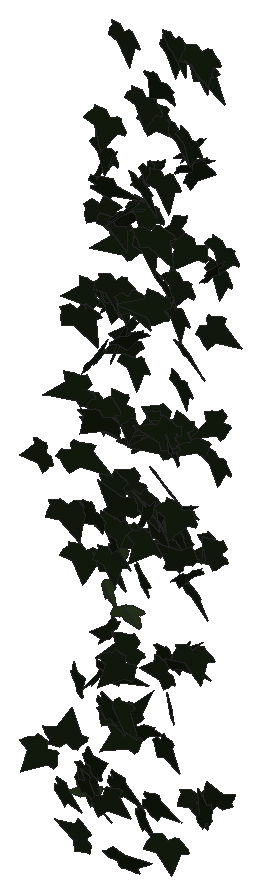
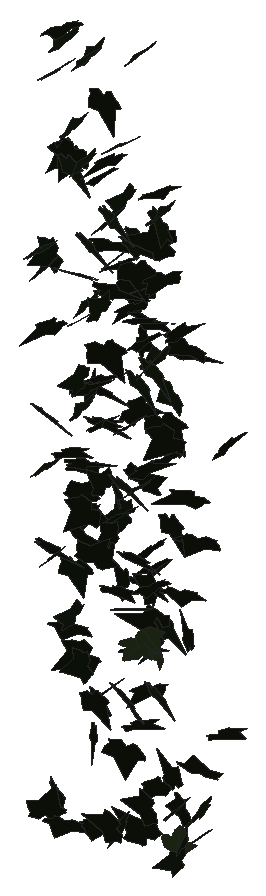
# SketchUp Ruby script. Lengths in inches.
U = 1.inch
M = Sketchup.active_model
def pt(a) = Geom::Point3d.new(a.map { |v| v * U })
def face(e, loops, mat)
  f = e.add_face(loops[0].map { |a| pt(a) })
  loops[1..].each { |l| e.add_face(l.map { |a| pt(a) }).erase! }
  f.material = f.back_material = mat if mat
  f
end
# faces: each face lists its corners as indices into pts; further lists are holes
def faces(e, pts, list, mat = nil) = list.each { |f| face(e, (f[0].is_a?(Array) ? f : [f]).map { |l| l.map { |i| pts[i] } }, mat) }
# xy, xz, yz: faces in a plane at the given z, y or x. An outline is a flat list of corners, or four numbers for a rectangle; further outlines are holes
def ring(l) = l.size == 4 ? [[l[0], l[1]], [l[2], l[1]], [l[2], l[3]], [l[0], l[3]]] : l.each_slice(2).to_a
def flat(e, list, mat, &to3) = list.each { |f| face(e, (f[0].is_a?(Array) ? f : [f]).map { |l| ring(l).map { |u, v| to3.(u, v) } }, mat) }
def xy(e, z, list, mat = nil) = flat(e, list, mat) { |x, y| [x, y, z] }
def xz(e, y, list, mat = nil) = flat(e, list, mat) { |x, z| [x, y, z] }
def yz(e, x, list, mat = nil) = flat(e, list, mat) { |y, z| [x, y, z] }
def lines(e, pts, list) = list.each { |a, b| e.add_line(pt(pts[a]), pt(pts[b])) }
# prism: a flat outline (further loops are holes) pulled along v
def prism(e, loops, v, mat = nil)
  f = face(e, loops, mat); d = Geom::Vector3d.new(v.map { |x| x * U })
  f.pushpull(f.normal.samedirection?(d) ? d.length : -d.length)
end
def box(e, o, s, mat = nil) = prism(e, [[o, [o[0] + s[0], o[1], o[2]], [o[0] + s[0], o[1] + s[1], o[2]], [o[0], o[1] + s[1], o[2]]]], [0, 0, s[2]], mat)
def at(x, y, z, deg = 0) = Geom::Transformation.translation(pt([x, y, z])) * Geom::Transformation.rotation(ORIGIN, Z_AXIS, deg.degrees)
def axes(o, x, y, z) = Geom::Transformation.new([*x, 0, *y, 0, *z, 0, *pt(o).to_a, 1])
def part(name) = M.definitions.add(name)
# library, detail: a bought-in or finely detailed component or shape, given as its bounding box
def library(name, o, s) = part(name).tap { |d| box(d.entities, o, s) }
def detail(e, o, s) = box(e.add_group.entities, o, s)
def put(e, d, t, mat = nil) = e.add_instance(d, t).tap { |i| i.material = mat if mat }
def group(e, t, mat = nil) = e.add_group.tap { |g| g.transformation = t; g.material = mat if mat }.entities
root = M.entities
M.materials.add("1026 AP 7946 SUNNY SIDE UP").color = [254, 231, 186]
M.materials.add("efeu1").color = [18, 25, 13]
M.materials.add("efeu2").color = [43, 57, 29]
c1 = part("ivyleaf_9")
p = [[1.54,2.16,1.25],[1.36,2.04,1.19],[-0.21,0.99,0.68],[-0.71,1.11,0.82],[-0.85,0.86,0.67],[-0.8,0.17,0.21],
  [-0.9,-0.01,0.1],[-0.67,-0.16,-0.02],[-0.08,-0.08,-0.05],[-0.03,-0.6,-0.4],[0.65,-0.88,-0.66],[0.83,-0.6,-0.49],
  [1.29,-0.42,-0.43],[1.8125,-0.07,-0.26],[1.21,0.44,0.15]]
faces(c1.entities,p,[[0,1,2,3,4,5,6,7,8,9,10,11,12,13,14]],"efeu1")
c2 = part("ivyleaf_10")
p = [[0,0.5,-0.03],[-0.0625,2.02,-0.43],[-0.19,2.01,-0.46],[-0.54,1.05,-0.29],[-0.52,0.625,-0.18],[-0.83,0.76,-0.28],
  [-1.16,0.64,-0.33],[-1.15,0.33,-0.24],[-0.77,-0.39,0.02],[-0.3,-0.51,0.16],[0.04,-0.48,0.23],[-0.02,2.01,-0.4375],
  [-0.06,2.01,-0.43],[0.04,-0.49,0.23],[0.67,-0.49,0.14],[1.38,0.36,-0.2],[1.375,0.51,-0.24],[0.81,0.65,-0.19],
  [0.62,0.59,-0.15],[0.6,1.09,-0.28],[0.5,1.23,-0.31]]
faces(c2.entities,p,[[0,1,2,3,4,5,6,7,8,9,10],[11,12,0,13,14,15,16,17,18,19,20]],"efeu2")
put(root,c1,axes([163.08,208.98,294.97],[-0.63448,0.06038,0.18044],[0.28089,0.01865,0.41828],[0.07528,0.43936,-0.03993]),"1026 AP 7946 SUNNY SIDE UP")
put(root,c1,axes([163.05,207.6,308.75],[0.10411,-0.32993,-0.29314],[0.18645,-0.26136,0.34135],[-0.65722,-0.12641,0.0504]),"1026 AP 7946 SUNNY SIDE UP")
put(root,c1,axes([162.83,211.46,318.29],[0.01182,-0.3708,-0.31812],[-0.03173,0.30622,-0.38012],[0.75597,0.01865,-0.01098]),"1026 AP 7946 SUNNY SIDE UP")
put(root,c1,axes([163.41,211.59,314.12],[-0.30515,0.40603,0.05346],[-0.04881,0.04011,-0.46325],[-0.64133,-0.19624,0.00982]),"1026 AP 7946 SUNNY SIDE UP")
put(root,c1,axes([162.99,211.79,322.14],[-0.27864,-0.43252,0.07285],[-0.00325,-0.07809,-0.48116],[0.68975,-0.17509,0.02716]),"1026 AP 7946 SUNNY SIDE UP")
put(root,c2,axes([163.2,210.21,292.14],[-0.48083,-0.24254,-0.10357],[-0.14812,-0.04045,0.40096],[-0.38447,0.31891,-0.02494]),"1026 AP 7946 SUNNY SIDE UP")
put(root,c2,axes([163.27,212.04,302.38],[-0.29776,-0.29187,0.20443],[-0.10278,-0.19419,-0.35667],[0.54686,-0.19542,0.04428]),"1026 AP 7946 SUNNY SIDE UP")
put(root,c1,axes([163.35,210.97,320.28],[0.00242,0.34278,0.33575],[-0.00805,0.32396,-0.3512],[-0.74157,-0.00239,0.00491]),"1026 AP 7946 SUNNY SIDE UP")
put(root,c1,axes([162.9375,209.25,305.52],[-0.29022,-0.31053,-0.2798],[0.24286,0.22181,-0.37051],[0.59955,-0.24016,0.01464]),"1026 AP 7946 SUNNY SIDE UP")
put(root,c1,axes([163.37,210.26,314.9],[-0.23905,-0.11298,0.40638],[-0.41094,-0.29853,-0.19328],[0.49866,-0.30017,0.03553]),"1026 AP 7946 SUNNY SIDE UP")
put(root,c1,axes([162.76,210.6,291.82],[0.50726,-0.26293,0.05987],[0.04536,-0.05876,-0.42818],[0.4215,0.32276,-0.02598]),"1026 AP 7946 SUNNY SIDE UP")
put(root,c1,axes([162.76,209.8125,307.75],[0.17736,-0.21342,-0.40951],[0.28851,0.39487,-0.16296],[0.64629,-0.1177,0.18513]),"1026 AP 7946 SUNNY SIDE UP")
put(root,c1,axes([162.98,210.26,292.22],[0.08539,-0.23069,0.33356],[0.07354,-0.32214,-0.24543],[0.62247,0.0697,-0.01676]),"1026 AP 7946 SUNNY SIDE UP")
put(root,c1,axes([163.07,211.49,314.72],[0.35675,-0.26779,-0.29291],[-0.23182,0.24388,-0.35833],[0.56683,0.26828,0.0378]),"1026 AP 7946 SUNNY SIDE UP")
put(root,c1,axes([163.04,211.53,320.92],[-0.05014,-0.38539,0.28073],[0.01768,-0.27585,-0.39897],[0.74395,-0.01941,0.0284]),"1026 AP 7946 SUNNY SIDE UP")
put(root,c1,axes([163.64,212.34,316.41],[-0.57045,-0.06544,0.26432],[-0.3141,-0.21888,-0.34928],[0.27415,-0.38695,0.14981]),"1026 AP 7946 SUNNY SIDE UP")
put(root,c1,axes([163.68,211.02,299.28],[-0.30723,0.33384,0.12004],[-0.11068,0.09153,-0.3977],[-0.54386,-0.20722,0.01313]),"1026 AP 7946 SUNNY SIDE UP")
put(root,c1,axes([163.15,208.4375,293.17],[0.44463,-0.23051,-0.25194],[-0.24259,0.19299,-0.37205],[0.46778,0.31919,0.04653]),"1026 AP 7946 SUNNY SIDE UP")
put(root,c1,axes([163.3125,209.875,303.32],[-0.43187,-0.29075,-0.16748],[0.22797,0.08302,-0.40895],[0.47018,-0.30731,0.04444]),"1026 AP 7946 SUNNY SIDE UP")
put(root,c1,axes([163.59,207.01,295.64],[-0.4412,-0.3086,0.17625],[-0.15128,-0.1457,-0.42978],[0.53519,-0.29558,0.02381]),"1026 AP 7946 SUNNY SIDE UP")
put(root,c1,axes([163.13,209.67,314.34],[-0.24854,-0.21835,-0.39324],[0.54926,0.18199,-0.25603],[0.41725,-0.36963,0.1028]),"1026 AP 7946 SUNNY SIDE UP")
put(root,c1,axes([163.35,210.96,309.73],[-0.14494,-0.43918,-0.01295],[0.00689,0.00938,-0.46224],[0.69072,-0.09225,0.00189]),"1026 AP 7946 SUNNY SIDE UP")
put(root,c2,axes([163.31,211.23,301.125],[-0.26702,0.10418,-0.35464],[0.30113,-0.29679,-0.19126],[-0.47975,-0.24427,0.07733]),"1026 AP 7946 SUNNY SIDE UP")
put(root,c1,axes([163.72,209.86,312.08],[-0.34317,0.30052,-0.30298],[-0.26093,0.245,0.38397],[0.60955,0.27406,-0.00621]),"1026 AP 7946 SUNNY SIDE UP")
put(root,c1,axes([163.81,211.77,309.38],[-0.00235,-0.29378,-0.33316],[-0.0092,-0.32168,0.30076],[-0.68499,0.00533,-0.0029]),"1026 AP 7946 SUNNY SIDE UP")
put(root,c1,axes([163.41,211.46,305.99],[0.13309,-0.39018,-0.16812],[-0.07608,0.15413,-0.41017],[0.65931,0.09655,-0.01339]),"1026 AP 7946 SUNNY SIDE UP")
put(root,c1,axes([163.31,211.68,317.8],[0.01726,-0.45722,0.01844],[0.1557,-0.01764,-0.46022],[0.70261,0.01514,0.10153]),"1026 AP 7946 SUNNY SIDE UP")
put(root,c1,axes([163.06,211.04,319.46],[0.51341,-0.02501,0.3479],[0.52361,-0.06252,-0.33668],[0.09787,0.46566,-0.02374]),"1026 AP 7946 SUNNY SIDE UP")
put(root,c1,axes([163.45,209.74,293.56],[0.23476,-0.40095,-0.05234],[-0.04958,0.04001,-0.44024],[0.63312,0.15181,-0.01506]),"1026 AP 7946 SUNNY SIDE UP")
put(root,c1,axes([164.04,212.22,305.73],[-0.62728,-0.02361,0.05639],[-0.08204,-0.04279,-0.40995],[0.04575,-0.40041,0.03811]),"1026 AP 7946 SUNNY SIDE UP")
put(root,c1,axes([163.49,211.3,314.13],[-0.09374,-0.32197,0.3189],[0.11807,-0.31686,-0.32458],[0.69432,0.01041,0.09825]),"1026 AP 7946 SUNNY SIDE UP")
put(root,c1,axes([163.6,211.41,304.14],[-0.14801,-0.42566,-0.04229],[0.01045,0.0381,-0.44888],[0.67198,-0.09435,-0.00234]),"1026 AP 7946 SUNNY SIDE UP")
put(root,c1,axes([163.99,212.07,312.21],[-0.10823,-0.1008,-0.4272],[0.10757,-0.41664,0.09033],[-0.66146,-0.05126,0.08459]),"1026 AP 7946 SUNNY SIDE UP")
put(root,c1,axes([163.72,212.03,308.7],[-0.03932,-0.39759,0.1504],[0.03084,-0.14943,-0.41032],[0.6665,-0.01654,0.02786]),"1026 AP 7946 SUNNY SIDE UP")
put(root,c1,axes([164.14,208.82,290.99],[-0.02009,-0.45157,-0.06725],[0.00847,-0.06288,0.46496],[-0.71681,0.01192,0.00738]),"1026 AP 7946 SUNNY SIDE UP")
put(root,c1,axes([163.53,209.36,293.33],[0.00174,-0.03834,-0.42669],[0.653,-0.01912,0.00285],[-0.03035,-0.41353,0.03699]),"1026 AP 7946 SUNNY SIDE UP")
put(root,c1,axes([164.15,211.55,318.28],[0.11189,0.38655,-0.2137],[-0.01882,-0.21058,-0.40544],[-0.69119,0.06831,-0.02355]),"1026 AP 7946 SUNNY SIDE UP")
put(root,c1,axes([164.35,211.28,313.09],[-0.27488,0.38905,0.09405],[-0.08026,0.07466,-0.43867],[-0.62242,-0.18144,0.01503]),"1026 AP 7946 SUNNY SIDE UP")
put(root,c1,axes([164.18,212.29,303.29],[-0.53516,-0.17468,0.15774],[-0.05763,-0.2293,-0.35248],[0.36172,-0.29496,0.17722]),"1026 AP 7946 SUNNY SIDE UP")
put(root,c1,axes([164.38,209.14,305.8],[0.25416,-0.01188,-0.41607],[-0.63241,-0.04563,-0.16474],[-0.05973,0.43256,-0.02625]),"1026 AP 7946 SUNNY SIDE UP")
put(root,c1,axes([163.98,211.28,314.93],[-0.01392,-0.45263,-0.03905],[-0.00901,0.03545,-0.46613],[0.71382,-0.00838,-0.00664]),"1026 AP 7946 SUNNY SIDE UP")
put(root,c1,axes([164.01,209.5,309.76],[0.63484,0.15416,0.03711],[0.07257,-0.02271,-0.44366],[-0.2378,0.40463,-0.03632]),"1026 AP 7946 SUNNY SIDE UP")
put(root,c1,axes([164.14,212.03,311.42],[-0.05628,-0.42003,0.092],[0.00801,-0.09241,-0.43462],[0.67596,-0.03388,0.01281]),"1026 AP 7946 SUNNY SIDE UP")
put(root,c1,axes([164.1875,210.73,315.58],[-0.40913,-0.24289,-0.26482],[0.41879,0.07292,-0.35016],[0.36346,-0.35743,0.10538]),"1026 AP 7946 SUNNY SIDE UP")
put(root,c1,axes([164.71,209.1875,310.21],[0.28814,0.15422,-0.41519],[-0.47548,-0.26781,-0.24825],[-0.48587,0.35354,-0.00329]),"1026 AP 7946 SUNNY SIDE UP")
put(root,c1,axes([164.22,209.12,294.18],[-0.03522,0.05051,0.43086],[0.26598,-0.38218,0.05468],[0.60617,0.17063,0.00104]),"1026 AP 7946 SUNNY SIDE UP")
put(root,c1,axes([164.07,210.66,303.51],[0.23508,-0.08895,-0.43349],[0.66107,-0.06116,0.16704],[-0.13882,-0.44187,0.0614]),"1026 AP 7946 SUNNY SIDE UP")
put(root,c1,axes([164.86,211.07,319.14],[-0.45746,0.20393,-0.28644],[0.1792,-0.28794,-0.34069],[-0.51327,-0.28229,0.13635]),"1026 AP 7946 SUNNY SIDE UP")
put(root,c1,axes([165.1,207.6,312.35],[-0.57636,-0.05835,0.25336],[-0.34857,-0.13508,-0.37368],[0.19199,-0.42042,0.08214]),"1026 AP 7946 SUNNY SIDE UP")
put(root,c1,axes([165.11,211.43,308.3125],[-0.38144,0.32202,0.09326],[-0.18356,0.02097,-0.40722],[-0.49208,-0.25744,0.07961]),"1026 AP 7946 SUNNY SIDE UP")
put(root,c1,axes([164.6875,212.17,318.47],[-0.2182,-0.4242,0.08992],[0.00588,-0.09534,-0.45913],[0.68173,-0.13495,0.03274]),"1026 AP 7946 SUNNY SIDE UP")
put(root,c2,axes([164.72,210.7,300.79],[-0.53763,-0.12286,-0.18286],[0.28097,0.02316,-0.37244],[0.18884,-0.38423,0.03353]),"1026 AP 7946 SUNNY SIDE UP")
put(root,c1,axes([164.6,209.51,303.7],[0.28805,-0.4025,-0.0996],[-0.02434,0.0965,-0.45427],[0.64961,0.1821,0.02714]),"1026 AP 7946 SUNNY SIDE UP")
put(root,c1,axes([164.71,210.62,327.17],[0.0333,-0.45718,0.13515],[0.02116,-0.13329,-0.47222],[0.74873,0.0241,0.00733]),"1026 AP 7946 SUNNY SIDE UP")
put(root,c1,axes([164.77,211.91,323.6],[-0.14609,-0.43549,0.15151],[0.06514,-0.15985,-0.45396],[0.72108,-0.07379,0.07171]),"1026 AP 7946 SUNNY SIDE UP")
put(root,c1,axes([165.32,211.94,320.45],[-0.48391,0.3282,-0.05919],[0.03113,-0.06259,-0.46297],[-0.5235,-0.30711,0.02718]),"1026 AP 7946 SUNNY SIDE UP")
put(root,c1,axes([165.15,211.75,303.64],[-0.55792,-0.19086,0.01111],[0.00901,-0.03562,-0.41378],[0.30055,-0.35323,0.03303]),"1026 AP 7946 SUNNY SIDE UP")
put(root,c1,axes([164.87,209.62,303.83],[-0.09044,-0.43096,0.00153],[0.00771,-0.00462,-0.4479],[0.67762,-0.05746,0.0053]),"1026 AP 7946 SUNNY SIDE UP")
put(root,c1,axes([165.45,211.93,314.39],[0.06435,0.35637,-0.28148],[-0.14711,-0.26363,-0.36749],[-0.69259,0.08911,0.05191]),"1026 AP 7946 SUNNY SIDE UP")
put(root,c1,axes([164.66,210.08,293.28],[0.1459,-0.02159,-0.45805],[0.69678,0.04641,0.09324],[0.06461,-0.45171,0.02879]),"1026 AP 7946 SUNNY SIDE UP")
put(root,c1,axes([164.91,211.95,320.4375],[0.35022,-0.37172,-0.1558],[-0.08929,0.13959,-0.44504],[0.62341,0.22882,0.02378]),"1026 AP 7946 SUNNY SIDE UP")
put(root,c1,axes([165.02,211.95,323.03],[0.25993,-0.28728,-0.36004],[-0.0603,0.36018,-0.32311],[0.70681,0.13638,0.10484]),"1026 AP 7946 SUNNY SIDE UP")
put(root,c1,axes([165.08,207.1,299.16],[-0.03593,0.07214,0.44543],[0.10127,-0.42729,0.07453],[0.68114,0.06734,0.01242]),"1026 AP 7946 SUNNY SIDE UP")
put(root,c1,axes([165.3,209.85,314],[-0.23077,0.10736,-0.41614],[0.44448,-0.29073,-0.18683],[-0.48536,-0.31729,0.02676]),"1026 AP 7946 SUNNY SIDE UP")
put(root,c1,axes([165.56,210.45,295.81],[0.39343,0.26893,-0.18285],[-0.17288,-0.14202,-0.37894],[-0.47766,0.27291,-0.01345]),"1026 AP 7946 SUNNY SIDE UP")
put(root,c1,axes([165.38,208.53,293.45],[0.09126,-0.18412,-0.4123],[-0.09453,0.39553,-0.19464],[0.68472,0.07915,0.02808]),"1026 AP 7946 SUNNY SIDE UP")
put(root,c1,axes([165.9,209.74,299.84],[-0.46094,-0.17309,0.30653],[-0.37609,-0.18044,-0.35079],[0.39112,-0.37749,0.02394]),"1026 AP 7946 SUNNY SIDE UP")
put(root,c1,axes([165.38,210.14,315.51],[0.11081,-0.35807,-0.25687],[-0.00152,0.2504,-0.37232],[0.68427,0.05854,0.04077]),"1026 AP 7946 SUNNY SIDE UP")
put(root,c1,axes([165.99,211.9375,298.58],[0.20573,0.06342,-0.39136],[-0.57795,-0.10058,-0.14815],[-0.1828,0.38935,0.02796]),"1026 AP 7946 SUNNY SIDE UP")
put(root,c1,axes([165.3,210.83,320.5],[0.30032,-0.41801,0.14631],[0.07043,-0.13819,-0.47398],[0.69182,0.19553,-0.01526]),"1026 AP 7946 SUNNY SIDE UP")
put(root,c1,axes([166.02,211.25,325.08],[0.39801,0.02477,-0.41906],[-0.6314,-0.06753,-0.26196],[-0.11065,0.47444,-0.01257]),"1026 AP 7946 SUNNY SIDE UP")
put(root,c1,axes([166.07,209.3,296.16],[-0.47088,-0.23784,0.2175],[-0.21549,-0.16721,-0.39279],[0.45282,-0.3269,0.03925]),"1026 AP 7946 SUNNY SIDE UP")
put(root,c1,axes([166.29,208.64,306.68],[0.09845,0.05486,0.44962],[-0.53682,0.28356,0.0154],[-0.43538,-0.33723,0.08267]),"1026 AP 7946 SUNNY SIDE UP")
put(root,c1,axes([165.6,210.6,306.32],[0.12777,-0.41433,-0.15494],[0.01872,0.15257,-0.43224],[0.69157,0.07242,0.04033]),"1026 AP 7946 SUNNY SIDE UP")
put(root,c1,axes([165.64,210.88,317.89],[0.08853,-0.45106,0.05295],[-0.00768,-0.05497,-0.46845],[0.71426,0.05532,-0.0116]),"1026 AP 7946 SUNNY SIDE UP")
put(root,c1,axes([166.14,207.4,299.87],[-0.39643,0.31865,-0.17145],[0.13161,-0.14792,-0.41872],[-0.5511,-0.26455,0.02334]),"1026 AP 7946 SUNNY SIDE UP")
put(root,c1,axes([165.54,210.48,306.25],[0.58423,-0.27681,0.04963],[0.03335,-0.05461,-0.47658],[0.44097,0.37087,-0.02971]),"1026 AP 7946 SUNNY SIDE UP")
put(root,c1,axes([165.78,208.6,297.63],[0.05609,-0.33006,-0.33384],[0.02028,0.32373,-0.3383],[0.72496,0.01648,0.03529]),"1026 AP 7946 SUNNY SIDE UP")
put(root,c1,axes([165.88,210.125,292.19],[0.41488,-0.28345,-0.21579],[-0.27649,0.11861,-0.39587],[0.47857,0.31425,-0.04164]),"1026 AP 7946 SUNNY SIDE UP")
put(root,c1,axes([165.72,211.23,305.4375],[-0.0134,-0.07881,0.44039],[0.21879,-0.40603,-0.07655],[0.64827,0.1354,0.03494]),"1026 AP 7946 SUNNY SIDE UP")
put(root,c1,axes([166.28,211.48,304.4],[0.39813,-0.0173,0.3663],[-0.53957,0.1047,0.25753],[-0.14954,-0.42385,0.04603]),"1026 AP 7946 SUNNY SIDE UP")
put(root,c1,axes([166.22,211.38,298.21],[0.13615,-0.37191,-0.22226],[0.10294,-0.20393,0.39188],[-0.66651,-0.10747,0.01512]),"1026 AP 7946 SUNNY SIDE UP")
put(root,c1,axes([165.74,210.3,302.89],[0.37048,-0.22499,-0.32373],[0.5298,-0.05792,0.30388],[-0.29436,-0.38744,0.13949]),"1026 AP 7946 SUNNY SIDE UP")
put(root,c1,axes([166.32,211.47,296.76],[0.30073,-0.13507,-0.37533],[-0.53754,0.13274,-0.2353],[0.28803,0.38876,-0.04725]),"1026 AP 7946 SUNNY SIDE UP")
put(root,c1,axes([166.07,209.33,296.9],[-0.28604,0.4282,0.13401],[0.093,-0.11354,0.47852],[0.6964,0.19104,-0.00886]),"1026 AP 7946 SUNNY SIDE UP")
put(root,c1,axes([165.89,211.63,315.75],[0.15856,-0.34295,0.30654],[0.13689,-0.28658,-0.36993],[0.70274,0.1332,0.0029]),"1026 AP 7946 SUNNY SIDE UP")
put(root,c1,axes([165.96,210.82,318.4],[-0.12895,-0.33638,-0.28983],[0.35448,0.21109,-0.32871],[0.58919,-0.20061,0.13433]),"1026 AP 7946 SUNNY SIDE UP")
put(root,c1,axes([165.78,210.88,292.35],[0.26897,-0.04643,-0.40331],[0.60213,0.11986,0.15853],[0.14563,-0.40982,0.08942]),"1026 AP 7946 SUNNY SIDE UP")
put(root,c1,axes([166.24,212.35,315.57],[-0.19117,-0.37624,0.19839],[0.00028,-0.20262,-0.40441],[0.66614,-0.10789,0.0571]),"1026 AP 7946 SUNNY SIDE UP")
put(root,c1,axes([166.8,211.52,318.58],[-0.52129,0.31362,0.00073],[-0.03516,-0.0252,-0.46901],[-0.49189,-0.33057,0.03276]),"1026 AP 7946 SUNNY SIDE UP")
put(root,c1,axes([166.89,212.01,308.73],[-0.40614,0.05913,0.33431],[-0.50487,-0.1378,-0.23846],[0.11653,-0.39092,0.132]),"1026 AP 7946 SUNNY SIDE UP")
put(root,c1,axes([166.75,210.78,310.19],[-0.67766,-0.08063,0.0688],[-0.08935,-0.05978,-0.44935],[0.13881,-0.43207,0.04666]),"1026 AP 7946 SUNNY SIDE UP")
put(root,c1,axes([166.18,210.82,305.01],[0.30718,-0.39599,0.00638],[-0.01586,-0.01438,-0.45469],[0.62259,0.19501,-0.01473]),"1026 AP 7946 SUNNY SIDE UP")
put(root,c1,axes([166.21,212.25,322.46],[0.15015,-0.43413,0.15498],[0.03518,-0.1516,-0.4587],[0.72288,0.09755,-0.00987]),"1026 AP 7946 SUNNY SIDE UP")
put(root,c1,axes([167.06,210.05,315.58],[-0.47786,0.0346,0.33159],[-0.5087,-0.02887,-0.31185],[-0.00418,-0.44158,0.04376]),"1026 AP 7946 SUNNY SIDE UP")
put(root,c1,axes([166.74,210.74,309.93],[-0.34619,-0.26883,0.28121],[-0.20023,-0.24743,-0.35631],[0.56999,-0.2502,0.04563]),"1026 AP 7946 SUNNY SIDE UP")
put(root,c1,axes([166.16,208.49,290.8],[0.04669,-0.13579,0.43197],[0.59492,-0.20913,-0.09842],[0.35772,0.36553,0.1073]),"1026 AP 7946 SUNNY SIDE UP")
put(root,c1,axes([166.92,209.25,306.34],[-0.04125,0.24589,0.35209],[-0.04497,0.3392,-0.25273],[-0.65872,-0.03856,-0.00479]),"1026 AP 7946 SUNNY SIDE UP")
put(root,c1,axes([166.4375,207.14,298.79],[0.44968,-0.33903,-0.18367],[-0.19207,0.12763,-0.45606],[0.56938,0.31081,-0.00879]),"1026 AP 7946 SUNNY SIDE UP")
put(root,c1,axes([166.41,211.75,326.9],[0.11692,-0.46136,0.101],[0.03327,-0.09855,-0.48197],[0.74176,0.07714,0.0057]),"1026 AP 7946 SUNNY SIDE UP")
put(root,c1,axes([166.83,208.19,315.1],[0.19753,0.42816,-0.05794],[-0.00841,-0.05956,-0.45987],[-0.67948,0.1252,-0.01115]),"1026 AP 7946 SUNNY SIDE UP")
put(root,c1,axes([166.14,207.66,299.8],[0.39914,-0.02688,0.37251],[0.54258,-0.11825,-0.25919],[0.17587,0.42581,-0.04577]),"1026 AP 7946 SUNNY SIDE UP")
put(root,c1,axes([166.36,212.18,312.73],[0.44777,-0.33344,0.07102],[0.04106,-0.07069,-0.45137],[0.53443,0.28481,-0.02483]),"1026 AP 7946 SUNNY SIDE UP")
put(root,c1,axes([166.5,212,311.25],[0.07964,-0.36974,0.21741],[0.04016,-0.21162,-0.38569],[0.66985,0.05664,-0.00273]),"1026 AP 7946 SUNNY SIDE UP")
put(root,c1,axes([166.9,212.32,317.45],[-0.63349,-0.21102,-0.00909],[0.13661,-0.15069,-0.43386],[0.30261,-0.37371,0.17684]),"1026 AP 7946 SUNNY SIDE UP")
put(root,c1,axes([166.41,210.74,307.32],[0.17792,-0.24469,0.3196],[0.2186,-0.27896,-0.27929],[0.58339,0.17915,0.00718]),"1026 AP 7946 SUNNY SIDE UP")
put(root,c1,axes([166.61,210.79,321.14],[-0.03333,-0.46495,0.00454],[-0.00738,-0.00684,-0.4795],[0.73113,-0.02126,-0.00464]),"1026 AP 7946 SUNNY SIDE UP")
put(root,c1,axes([167.2,211.98,322.13],[-0.3109,0.41385,-0.00618],[-0.02285,-0.01618,-0.47215],[-0.65048,-0.19724,0.01954]),"1026 AP 7946 SUNNY SIDE UP")
put(root,c1,axes([166.59,211.34,326.76],[0.05747,-0.39343,0.275],[0.0251,-0.2688,-0.40855],[0.74914,0.03919,-0.00741]),"1026 AP 7946 SUNNY SIDE UP")
put(root,c1,axes([167.41,210.84,304.5625],[-0.05629,0.07804,0.45259],[-0.46047,0.32784,-0.08274],[-0.52846,-0.29397,0.02389]),"1026 AP 7946 SUNNY SIDE UP")
put(root,c1,axes([166.98,211.15,299.27],[0.20503,0.1572,0.39977],[0.33156,0.3254,-0.20737],[-0.56726,0.24701,0.02329]),"1026 AP 7946 SUNNY SIDE UP")
put(root,c1,axes([166.82,212.1,301.96],[0.32293,-0.37694,0.12991],[0.07648,-0.11946,-0.44269],[0.62137,0.2106,-0.01303]),"1026 AP 7946 SUNNY SIDE UP")
put(root,c1,axes([167.46,211.91,309],[-0.4603,-0.24105,0.18465],[-0.1892,-0.13729,-0.3905],[0.43418,-0.31538,0.02559]),"1026 AP 7946 SUNNY SIDE UP")
put(root,c1,axes([167.12,210.77,306.07],[0.39678,0.31037,0.17035],[0.19726,0.10838,-0.41052],[-0.5152,0.28052,-0.02598]),"1026 AP 7946 SUNNY SIDE UP")
put(root,c1,axes([167.61,206.9375,300.99],[-0.68277,-0.09128,-0.04141],[0.07478,-0.03427,-0.45514],[0.13748,-0.43468,0.0419]),"1026 AP 7946 SUNNY SIDE UP")
put(root,c1,axes([167.13,210.93,315.22],[0.07133,-0.42677,0.2093],[0.00587,-0.2062,-0.44302],[0.74484,0.04249,-0.01655]),"1026 AP 7946 SUNNY SIDE UP")
put(root,c1,axes([167.32,212.05,292.59],[-0.29495,-0.27141,-0.25758],[0.259,0.18748,-0.33795],[0.5174,-0.24856,0.02234]),"1026 AP 7946 SUNNY SIDE UP")
put(root,c1,axes([167.76,210.83,303.41],[0.04897,0.39609,-0.10533],[-0.01088,-0.10427,-0.40992],[-0.64404,0.03188,-0.00108]),"1026 AP 7946 SUNNY SIDE UP")
put(root,c1,axes([167.47,209.93,291.49],[-0.36109,-0.3017,-0.21132],[0.22738,0.14505,-0.38897],[0.52502,-0.27032,0.02312]),"1026 AP 7946 SUNNY SIDE UP")
put(root,c1,axes([167.31,210.46,305.52],[0.36382,-0.3832,0.0391],[0.00061,-0.04658,-0.46078],[0.60584,0.23016,-0.02301]),"1026 AP 7946 SUNNY SIDE UP")
put(root,c1,axes([167.34,210.6,299.41],[0.62699,0.12828,0.13611],[0.21581,0.0005,-0.42958],[-0.19183,0.41984,-0.0384]),"1026 AP 7946 SUNNY SIDE UP")
put(root,c1,axes([167.7,211.02,322],[0.32566,0.4024,0.09149],[0.09744,0.06527,-0.46515],[-0.63981,0.21476,-0.02427]),"1026 AP 7946 SUNNY SIDE UP")
put(root,c1,axes([168.24,209.1,310.39],[-0.67245,0.09479,0.16577],[-0.267,-0.0332,-0.44647],[-0.12047,-0.45553,0.06424]),"1026 AP 7946 SUNNY SIDE UP")
put(root,c1,axes([167.67,211.15,323.04],[-0.03181,-0.36709,0.28697],[0.02364,-0.28128,-0.37957],[0.72618,-0.00692,0.02493]),"1026 AP 7946 SUNNY SIDE UP")
put(root,c1,axes([168.32,209.16,310.61],[-0.34758,0.06106,0.39759],[-0.52102,-0.26365,-0.15422],[0.32459,-0.35781,0.1782]),"1026 AP 7946 SUNNY SIDE UP")
put(root,c1,axes([167.96,212.29,304.17],[-0.16376,-0.28358,0.28368],[-0.10925,-0.26889,-0.3121],[0.61366,-0.12355,0.02015]),"1026 AP 7946 SUNNY SIDE UP")
put(root,c1,axes([167.66,211.9,326.09],[0.24085,-0.44336,-0.09554],[0.04129,0.10381,-0.47896],[0.71023,0.14432,0.06024]),"1026 AP 7946 SUNNY SIDE UP")
put(root,c1,axes([168.36,209.95,310.52],[-0.29001,0.0476,0.39072],[-0.49556,-0.25676,-0.12628],[0.33935,-0.33427,0.14949]),"1026 AP 7946 SUNNY SIDE UP")
put(root,c1,axes([168.05,210.87,321.92],[0.00679,0.0436,-0.47483],[-0.31041,0.41737,0.04119],[0.6589,0.19617,0.0243]),"1026 AP 7946 SUNNY SIDE UP")
put(root,c1,axes([167.78,209.19,296.5],[-0.09517,-0.03915,-0.43407],[0.66401,0.01807,-0.06415],[0.03699,-0.42507,0.03474]),"1026 AP 7946 SUNNY SIDE UP")
put(root,c1,axes([168.73,211.63,304.3125],[-0.61456,0.10518,0.17378],[-0.27024,0.00559,-0.41526],[-0.15549,-0.42542,0.03486]),"1026 AP 7946 SUNNY SIDE UP")
put(root,c1,axes([168.32,211.97,292.58],[0.3582,0.16092,0.31804],[-0.48701,-0.07247,0.27476],[0.24716,-0.37601,0.08046]),"1026 AP 7946 SUNNY SIDE UP")
put(root,c1,axes([168.16,212.28,308.15],[-0.0734,-0.37848,0.19738],[0.04231,-0.19715,-0.39123],[0.66722,-0.02913,0.04652]),"1026 AP 7946 SUNNY SIDE UP")
put(root,c1,axes([168.11,211.77,314.45],[0.24723,-0.18942,-0.42186],[-0.10082,0.41878,-0.22307],[0.70069,0.12709,0.11675]),"1026 AP 7946 SUNNY SIDE UP")
put(root,c1,axes([168.04,211.13,326.83],[0.10242,-0.43725,0.18291],[0.09818,-0.17219,-0.4551],[0.73701,0.0837,0.03521]),"1026 AP 7946 SUNNY SIDE UP")
put(root,c1,axes([168.4,209.59,307.07],[-0.43093,-0.35034,0.00821],[0.02448,-0.0248,-0.4575],[0.55056,-0.27312,0.02677]),"1026 AP 7946 SUNNY SIDE UP")
put(root,c1,axes([168.29,209.27,310],[-0.10462,-0.07872,0.44592],[-0.02615,-0.43746,-0.08707],[0.69198,-0.02843,0.06413]),"1026 AP 7946 SUNNY SIDE UP")
put(root,c1,axes([168.83,211.68,310.3125],[-0.65605,0.11652,-0.01458],[0.00516,-0.04308,-0.44456],[-0.18462,-0.41526,0.03938]),"1026 AP 7946 SUNNY SIDE UP")
put(root,c1,axes([168.32,211.03,327.32],[-0.13667,-0.46329,-0.07902],[0.01878,0.07312,-0.48517],[0.73749,-0.08772,-0.00229]),"1026 AP 7946 SUNNY SIDE UP")
put(root,c1,axes([168.8,210.67,292.61],[0.04138,0.02595,0.45177],[-0.13171,0.43141,-0.01861],[-0.67785,-0.08224,0.03119]),"1026 AP 7946 SUNNY SIDE UP")
put(root,c1,axes([168.37,210.43,300.28],[-0.31715,-0.28898,-0.24033],[0.28565,0.15266,-0.35826],[0.50749,-0.26652,0.05146]),"1026 AP 7946 SUNNY SIDE UP")
put(root,c1,axes([168.4,212.41,317.8125],[-0.16433,-0.37857,0.23043],[0.0442,-0.23733,-0.39787],[0.69172,-0.07477,0.08017]),"1026 AP 7946 SUNNY SIDE UP")
put(root,c1,axes([168.375,212.15,316.88],[-0.02057,-0.39083,0.21568],[-0.00511,-0.21158,-0.40408],[0.69879,-0.01305,0.00339]),"1026 AP 7946 SUNNY SIDE UP")
put(root,c1,axes([168.53,211.19,317.17],[0.23331,0.21685,0.38307],[0.2963,0.31946,-0.26841],[-0.60669,0.23941,0.01623]),"1026 AP 7946 SUNNY SIDE UP")
put(root,c1,axes([169.04,208.96,305.1875],[0.1185,0.07943,0.42373],[-0.61919,-0.12779,0.09911],[0.22264,-0.39768,0.05012]),"1026 AP 7946 SUNNY SIDE UP")
